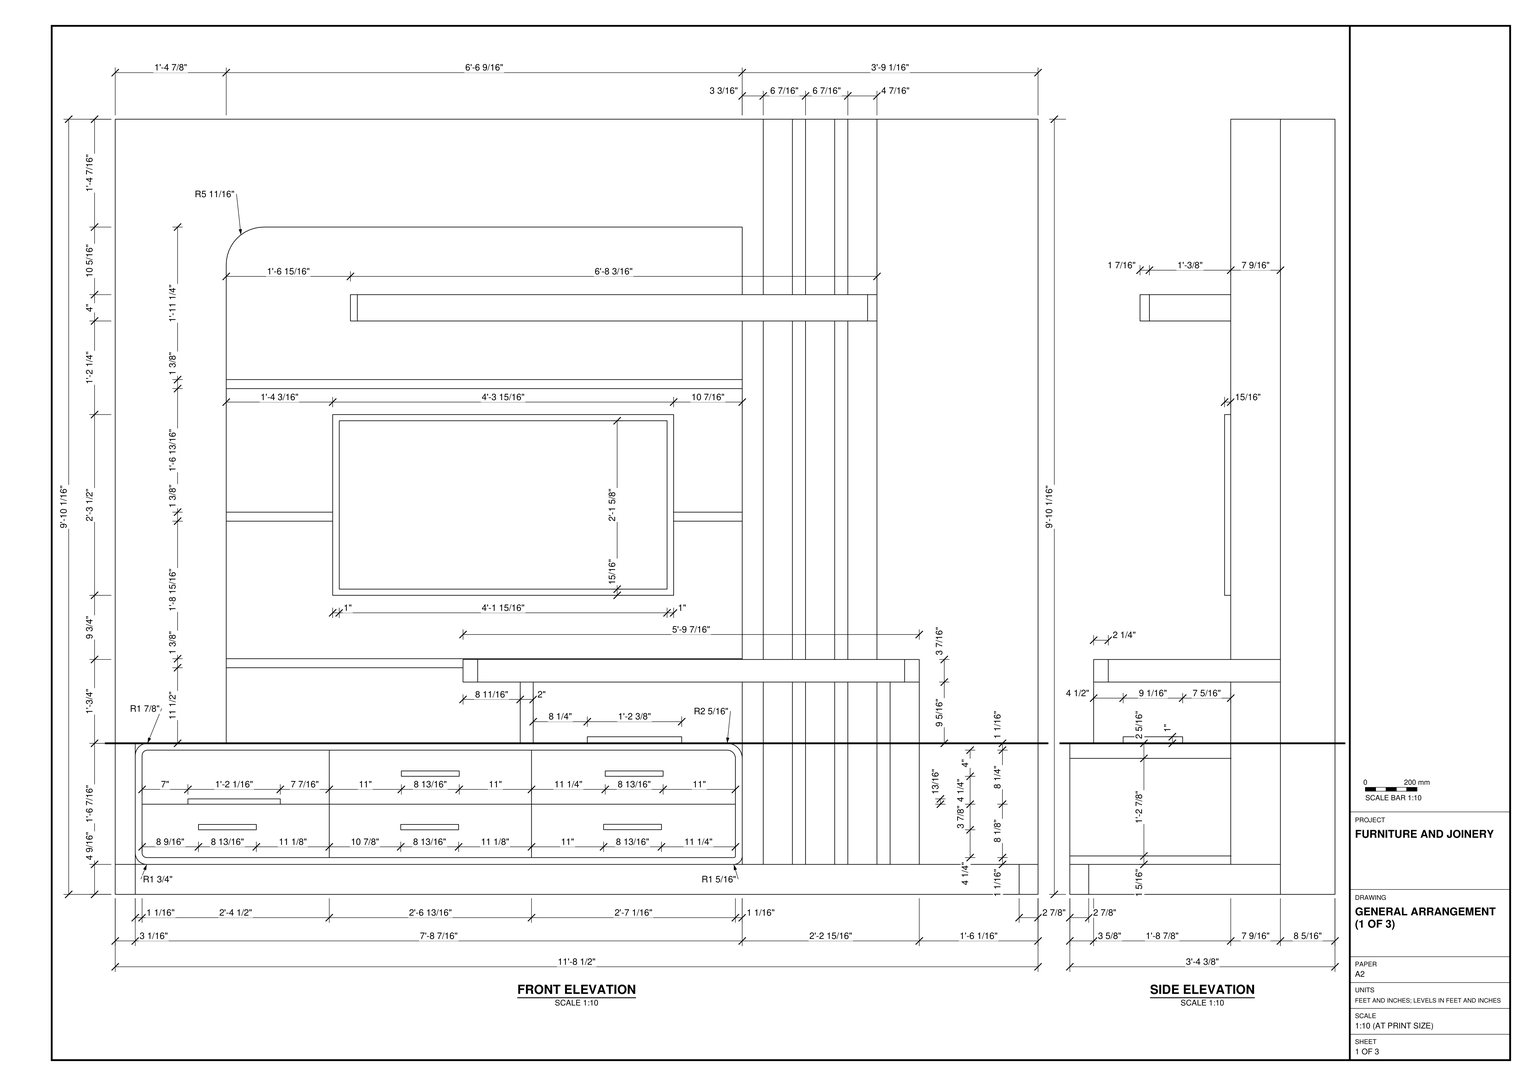
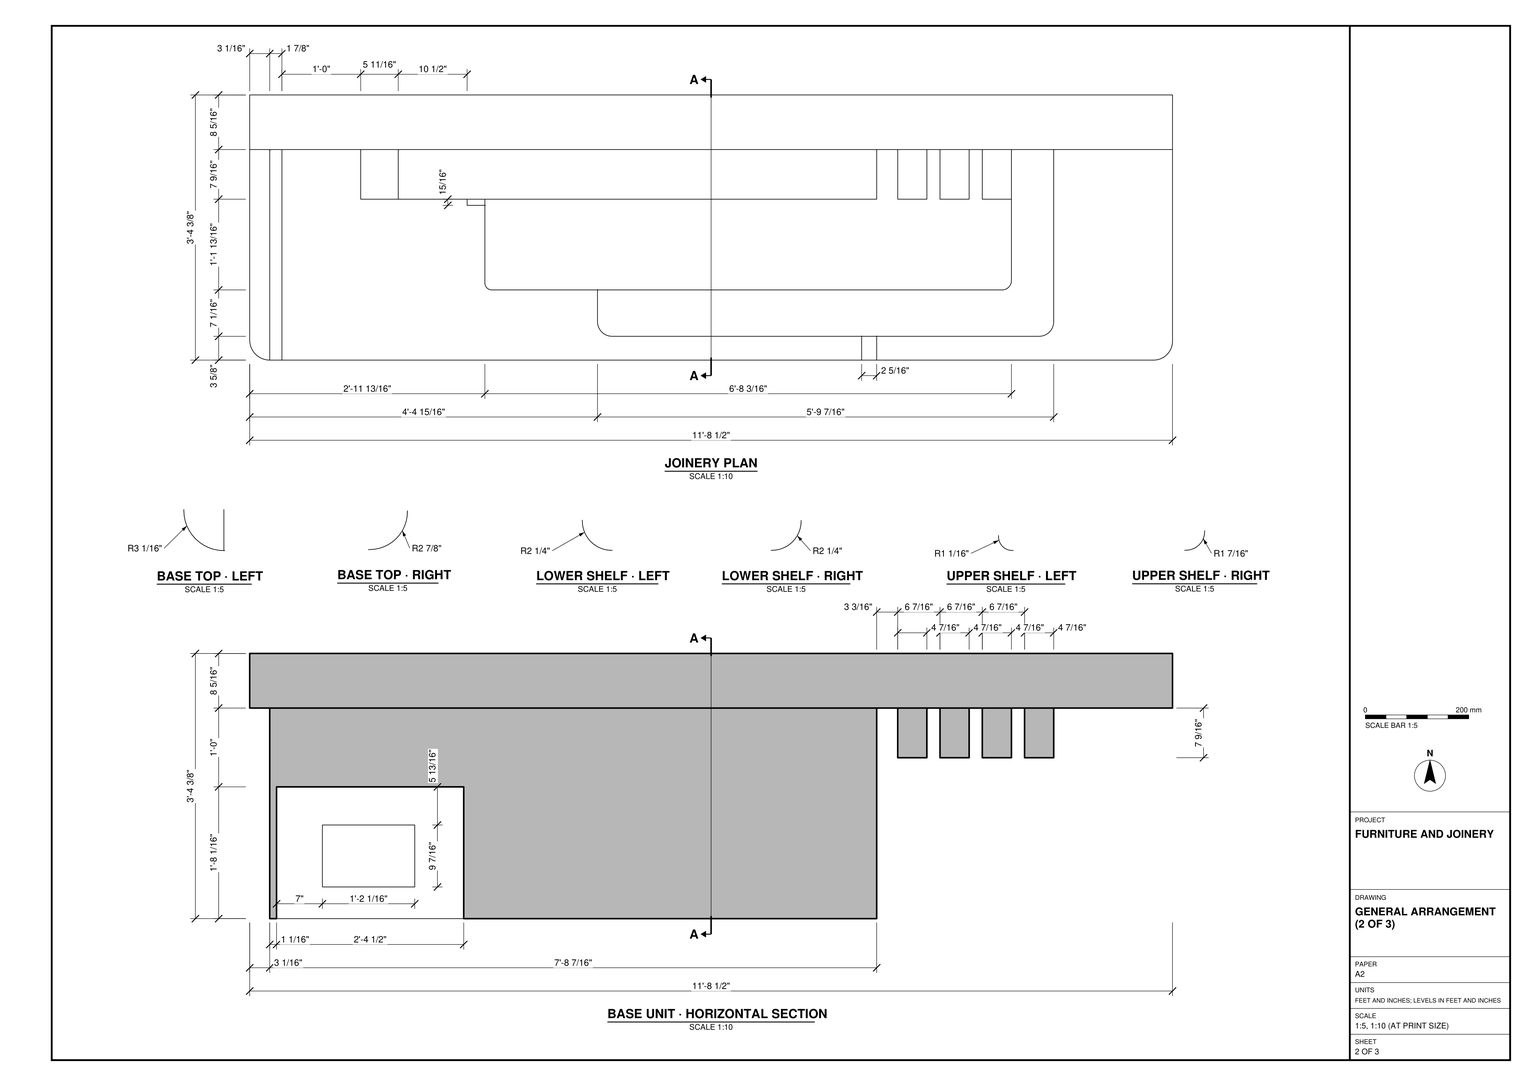
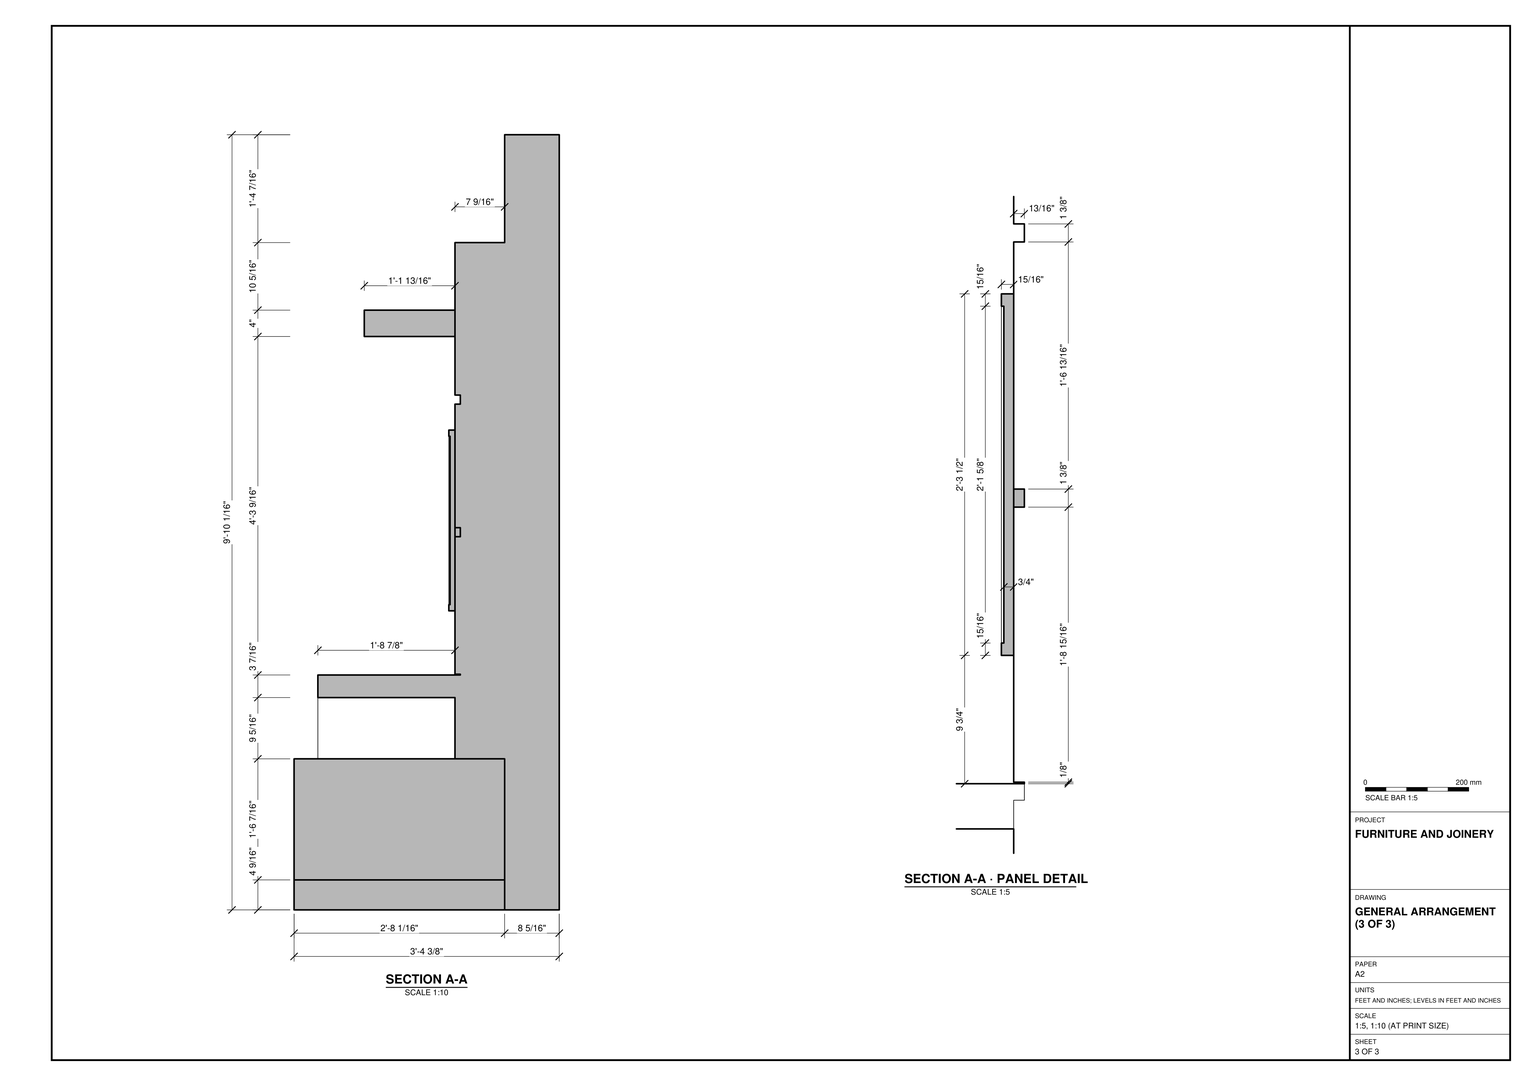
Build the media wall in SketchUp from task_files/diagram_01.pdf. Work in feet and inches. Use ±0'-0" as the floor datum and make the complete assembly 11'-8 1/2" wide, 3'-4 3/8" deep and 9'-10" high, including the rear wall.

Use the front elevation to lay out the raised backing panel, the framed screen, the narrow vertical strips on the right and the low storage cabinet on the left. Round the upper-left corner of the backing panel and form the horizontal grooves across its face. Set the screen between the two shelves. The upper shelf starts farther left, while the lower shelf extends farther right and projects farther forward. Use the plan and corner details to shape the front corners of the shelves and base top. Follow section A-A for the thickness of the rear wall, the changes in face depth and the clear space between the lower shelf and cabinet. Model the cabinet surround, bay divisions and pulls as shown in elevation.

Keep the rear wall and distinct joinery pieces in separate groups or components, and use components for repeated parts. Any decor or loose items shown may be represented by suitable library components. Save one SketchUp model as output_files/media_wall_with_base_storage_and_staggered_shelves.skp.

# SketchUp Ruby script. Lengths in inches.
U = 1.inch
M = Sketchup.active_model
def pt(a) = Geom::Point3d.new(a.map { |v| v * U })
def face(e, loops, mat)
  f = e.add_face(loops[0].map { |a| pt(a) })
  loops[1..].each { |l| e.add_face(l.map { |a| pt(a) }).erase! }
  f.material = f.back_material = mat if mat
  f
end
# faces: each face lists its corners as indices into pts; further lists are holes
def faces(e, pts, list, mat = nil) = list.each { |f| face(e, (f[0].is_a?(Array) ? f : [f]).map { |l| l.map { |i| pts[i] } }, mat) }
# xy, xz, yz: faces in a plane at the given z, y or x. An outline is a flat list of corners, or four numbers for a rectangle; further outlines are holes
def ring(l) = l.size == 4 ? [[l[0], l[1]], [l[2], l[1]], [l[2], l[3]], [l[0], l[3]]] : l.each_slice(2).to_a
def flat(e, list, mat, &to3) = list.each { |f| face(e, (f[0].is_a?(Array) ? f : [f]).map { |l| ring(l).map { |u, v| to3.(u, v) } }, mat) }
def xy(e, z, list, mat = nil) = flat(e, list, mat) { |x, y| [x, y, z] }
def xz(e, y, list, mat = nil) = flat(e, list, mat) { |x, z| [x, y, z] }
def yz(e, x, list, mat = nil) = flat(e, list, mat) { |y, z| [x, y, z] }
def lines(e, pts, list) = list.each { |a, b| e.add_line(pt(pts[a]), pt(pts[b])) }
# prism: a flat outline (further loops are holes) pulled along v
def prism(e, loops, v, mat = nil)
  f = face(e, loops, mat); d = Geom::Vector3d.new(v.map { |x| x * U })
  f.pushpull(f.normal.samedirection?(d) ? d.length : -d.length)
end
def box(e, o, s, mat = nil) = prism(e, [[o, [o[0] + s[0], o[1], o[2]], [o[0] + s[0], o[1] + s[1], o[2]], [o[0], o[1] + s[1], o[2]]]], [0, 0, s[2]], mat)
def at(x, y, z, deg = 0) = Geom::Transformation.translation(pt([x, y, z])) * Geom::Transformation.rotation(ORIGIN, Z_AXIS, deg.degrees)
def axes(o, x, y, z) = Geom::Transformation.new([*x, 0, *y, 0, *z, 0, *pt(o).to_a, 1])
def part(name) = M.definitions.add(name)
# library, detail: a bought-in or finely detailed component or shape, given as its bounding box
def library(name, o, s) = part(name).tap { |d| box(d.entities, o, s) }
def detail(e, o, s) = box(e.add_group.entities, o, s)
def put(e, d, t, mat = nil) = e.add_instance(d, t).tap { |i| i.material = mat if mat }
def group(e, t, mat = nil) = e.add_group.tap { |g| g.transformation = t; g.material = mat if mat }.entities
root = M.entities
M.materials.add("[Carrera Marble]").color = [177, 149, 108]
M.materials.add("[Color C02]").color = [255, 204, 153]
M.materials.add("[Color D01]").color = [255, 242, 204]
M.materials.add("[Color M09]").color = [0, 0, 0]
M.materials.add("[Wood Cherry Original]").color = [152, 86, 42]
xy(root,18.35,[[3.05,0,2.65,0.03,2.26,0.1,1.88,0.23,1.53,0.41,1.19,0.63,0.89,0.89,0.63,1.19,0.41,1.53,0.23,1.88,0.1,2.26,0.03,2.65,0,3.05,0,32.0625,140.5,32.0625,140.5,2.88,140.48,2.5,140.4,2.13,140.28,1.78,140.11,1.44,139.9,1.125,139.66,0.84,139.375,0.6,139.06,0.39,138.72,0.22,138.37,0.1,138,0.02,137.62,0],[0,32.0625,140.5,40.375]])
xy(root,22.91,[[3.05,0,3.05,32.0625,0,32.0625,0,3.05,0.03,2.65,0.1,2.26,0.23,1.88,0.41,1.53,0.63,1.19,0.89,0.89,1.19,0.63,1.53,0.41,1.88,0.23,2.26,0.1,2.65,0.03],[3.05,0,4.8,31.9375],[4.8,0,4.8,31.9375,3.05,31.9375,3.05,32.0625,94.17,32.0625,94.17,0],[94.17,0,95.46,32.0625],[98.66,24.5,103.1,32.0625],
  [105.1,24.5,109.54,32.0625],[111.54,24.5,115.98,32.0625],[117.98,24.5,122.41,32.0625]])
xy(root,22.91,[[95.46,0,137.62,0,138,0.02,138.37,0.1,138.72,0.22,139.06,0.39,139.375,0.6,139.66,0.84,139.9,1.125,140.11,1.44,140.28,1.78,140.4,2.13,140.48,2.5,140.5,2.88,140.5,32.0625,122.41,32.0625,122.41,24.5,117.98,24.5,117.98,32.0625,115.98,32.0625,115.98,24.5,111.54,24.5,111.54,32.0625,109.54,32.0625,109.54,24.5,105.1,24.5,105.1,32.0625,103.1,32.0625,103.1,24.5,98.66,24.5,98.66,32.0625,95.46,32.0625]],"[Color D01]")
xy(root,32.08,[[[4.09,0,32.59,20.0625],[11.07,4.82,25.13,14.26]]],"[Color D01]")
xy(root,32.89,[[11.07,4.82,25.13,14.26]],"[Color M09]")
xy(root,40.3125,[[4.91,0,32.59,20.0625]],"[Color D01]")
xy(root,41.35,[[16.9,24.5,93.17,32.0625],[93.17,24.5,95.46,32.0625]])
xy(root,41.35,[[[4.91,0,93.17,0,93.17,24.5,63.64,24.5,63.64,3.625,61.66,3.625,61.66,24.5,16.9,24.5,16.9,32.0625,4.91,32.0625],[71.87,8.12,86.25,17.18]]],"[Color D01]")
xy(root,42.35,[[71.87,8.12,86.25,17.18]],"[Color M09]")
xy(root,50.67,[[55.18,3.625,54.89,3.64,54.61,3.7,54.33,3.79,54.07,3.92,53.83,4.09,53.61,4.28,53.41,4.5,53.25,4.74,53.12,5,53.03,5.28,52.97,5.5625,52.95,5.86,52.95,24.5,61.66,24.5,61.66,3.625],[61.66,3.625,63.64,24.5],[98.66,24.5,103.1,26.8125],[105.1,24.5,109.54,26.8125],[111.54,24.5,115.98,26.8125],
  [117.98,24.5,122.41,32.0625]])
xy(root,50.67,[[63.64,3.625,63.64,24.5,95.46,24.5,95.46,32.0625,98.66,32.0625,98.66,24.5,103.1,24.5,103.1,32.0625,105.1,32.0625,105.1,24.5,109.54,24.5,109.54,32.0625,111.54,32.0625,111.54,24.5,115.98,24.5,115.98,32.0625,117.98,32.0625,117.98,24.5,122.41,24.5,122.41,5.86,122.39,5.5625,122.34,5.28,122.24,5,122.11,4.74,121.95,4.5,121.76,4.28,121.54,4.09,121.3,3.92,121.04,3.79,120.76,3.7,120.47,3.64,120.18,3.625]],"[Color D01]")
xy(root,52.86,[[16.9,24.5,52.95,25.3125]])
xy(root,54.12,[[98.66,24.5,103.1,26.8125],[105.1,24.5,109.54,26.8125],[111.54,24.5,115.98,26.8125]])
xy(root,54.12,[[55.18,3.625,120.18,3.625,120.47,3.64,120.76,3.7,121.04,3.79,121.3,3.92,121.54,4.09,121.76,4.28,121.95,4.5,122.11,4.74,122.24,5,122.34,5.28,122.39,5.5625,122.41,5.86,122.41,32.0625,115.98,32.0625,115.98,24.5,111.54,24.5,111.54,32.0625,109.54,32.0625,109.54,24.5,105.1,24.5,105.1,32.0625,103.1,32.0625,103.1,24.5,98.66,24.5,98.66,32.0625,95.46,32.0625,95.46,25.3125,52.95,25.3125,52.95,5.86,52.97,5.5625,53.03,5.28,53.12,5,53.25,4.74,53.41,4.5,53.61,4.28,53.83,4.09,54.07,3.92,54.33,3.79,54.61,3.7,54.89,3.64]],"[Color D01]")
xy(root,54.23,[[16.9,24.5,95.46,25.3125]])
xy(root,75.17,[[16.9,24.5,95.46,25.3125]])
xy(root,76.55,[[16.9,24.5,95.46,25.3125]])
xy(root,95.36,[[16.9,24.5,95.46,25.3125]])
xy(root,96.73,[[16.9,24.5,95.46,25.3125]])
xy(root,105.65,[[36.86,10.6875,36.72,10.7,36.59,10.72,36.46,10.77,36.33,10.83,36.22,10.91,36.12,11,36.03,11.1,35.95,11.21,35.89,11.34,35.84,11.47,35.82,11.6,35.81,11.74,35.81,24.5,95.46,24.5,95.46,32.0625,98.66,32.0625,98.66,24.5,103.1,24.5,103.1,35.125,105.1,35.125,105.1,24.5,109.54,24.5,109.54,35.125,111.54,35.125,111.54,24.5,115.98,24.5,115.98,12.11,115.96,11.93,115.93,11.74,115.87,11.57,115.78,11.4,115.68,11.25,115.56,11.11,115.42,10.98,115.26,10.88,115.1,10.8,114.92,10.74,114.74,10.7,114.55,10.6875]])
xy(root,109.67,[[36.86,10.6875,114.55,10.6875,114.74,10.7,114.92,10.74,115.1,10.8,115.26,10.88,115.42,10.98,115.56,11.11,115.68,11.25,115.78,11.4,115.87,11.57,115.93,11.74,115.96,11.93,115.98,12.11,115.98,24.5,111.54,24.5,111.54,35.125,109.54,35.125,109.54,24.5,105.1,24.5,105.1,35.125,103.1,35.125,103.1,24.5,98.66,24.5,98.66,32.0625,95.46,32.0625,95.46,24.5,35.81,24.5,35.81,11.74,35.82,11.6,35.84,11.47,35.89,11.34,35.95,11.21,36.03,11.1,36.12,11,36.22,10.91,36.33,10.83,36.46,10.77,36.59,10.72,36.72,10.7]],"[Color D01]")
xy(root,119.95,[[22.62,24.5,95.46,32.0625]],"[Color D01]")
xy(root,136.38,[[0,32.0625,140.5,40.375]],"[Color D01]")
xy(root,136.38,[[98.66,24.5,103.1,32.0625],[105.1,24.5,109.54,32.0625],[111.54,24.5,115.98,32.0625]],"[Wood Cherry Original]")
xz(root,0,[[3.05,18.35,137.62,22.91],[[4.8,22.91,94.17,22.91,94.34,22.92,94.51,22.96,94.67,23.01,94.82,23.08,94.96,23.18,95.08,23.29,95.2,23.42,95.29,23.56,95.36,23.71,95.42,23.87,95.45,24.03,95.46,24.2,95.46,39.06,95.44,39.36,95.38,39.65,95.29,39.94,95.15,40.2,94.99,40.45,94.79,40.68,94.56,40.875,94.32,41.04,94.05,41.18,93.76,41.27,93.47,41.33,93.17,41.35,4.91,41.35,4.67,41.33,4.43,41.29,4.2,41.21,3.98,41.1,3.78,40.97,3.59,40.81,3.43,40.62,3.3,40.42,3.19,40.2,3.11,39.97,3.07,39.73,3.05,39.49,3.05,24.66,3.07,24.43,3.11,24.21,3.18,23.99,3.28,23.79,3.41,23.6,3.5625,23.42,3.73,23.27,3.92,23.15,4.13,23.05,4.35,22.97,4.57,22.93],[4.8,23.95,4.62,23.97,4.53,24,4.44,24.04,4.3,24.16,4.23,24.23,4.18,24.31,4.14,24.39,4.11,24.48,4.09,24.57,4.09,39.6,4.12,39.7,4.15,39.81,4.2,39.9,4.26,39.99,4.33,40.07,4.41,40.14,4.5,40.2,4.59,40.25,4.7,40.28,4.8,40.31,4.91,40.3125,93.17,40.3125,93.33,40.3,93.49,40.27,93.65,40.22,93.8,40.14,93.93,40.05,94.06,39.95,94.17,39.82,94.26,39.69,94.33,39.54,94.38,39.38,94.41,39.22,94.42,39.06,94.42,24.14,94.41,24.1,94.39,24.07,94.37,24.05,94.35,24.02,94.33,24,94.3,23.98,94.21,23.95]]],"[Color D01]")
xz(root,0,[[12.67,28.18,21.48,28.99],[43.47,28.18,52.28,28.99],[74.35,28.2,83.17,29.01],[43.5625,36.33,52.375,37.14],[74.61,36.33,83.42,37.14]],"[Color M09]")
xz(root,0,[[[4.8,23.95,32.59,23.95,32.59,32.08,4.09,32.08,4.09,24.57,4.11,24.48,4.14,24.39,4.18,24.31,4.23,24.23,4.3,24.16,4.44,24.04,4.53,24,4.62,23.97],[12.67,28.18,21.48,28.99]],[[32.59,23.95,63.38,32.08],[43.47,28.18,52.28,28.99]],[[63.38,23.95,94.21,23.95,94.3,23.98,94.33,24,94.35,24.02,94.37,24.05,94.39,24.07,94.41,24.1,94.42,24.14,94.42,32.08,63.38,32.08],[74.35,28.2,83.17,29.01]],[[32.59,32.08,63.38,40.3125],[43.5625,36.33,52.375,37.14]],[[63.38,32.08,94.42,32.08,94.42,39.06,94.41,39.22,94.38,39.38,94.33,39.54,94.26,39.69,94.17,39.82,94.06,39.95,93.93,40.05,93.8,40.14,93.65,40.22,93.49,40.27,93.33,40.3,93.17,40.3125,63.38,40.3125],[74.61,36.33,83.42,37.14]]],"[Wood Cherry Original]")
xz(root,3.625,[[61.66,41.35,63.64,50.67],[55.18,50.67,120.18,54.12]],"[Color D01]")
xz(root,4.82,[[11.07,32.08,25.13,32.89]],"[Color M09]")
xz(root,8.12,[[71.87,41.35,86.25,42.35]],"[Color M09]")
xz(root,10.6875,[[36.86,105.65,114.55,109.67]],"[Color D01]")
xz(root,14.26,[[11.07,32.08,25.13,32.89]])
xz(root,17.18,[[71.87,41.35,86.25,42.35]])
xz(root,20.0625,[[4.09,32.08,32.59,32.08,32.59,40.3125,4.91,40.3125,4.8,40.31,4.7,40.28,4.59,40.25,4.5,40.2,4.41,40.14,4.33,40.07,4.26,39.99,4.2,39.9,4.15,39.81,4.12,39.7,4.09,39.6]],"[Color D01]")
xz(root,24.5,[[61.66,41.35,63.64,50.67],[35.81,105.65,95.46,109.67],[98.66,105.65,103.1,109.67],[105.1,105.65,109.54,109.67],[111.54,105.65,115.98,109.67]])
xz(root,24.5,[[16.9,41.35,61.66,41.35,61.66,50.67,52.95,50.67,52.95,52.86,16.9,52.86],[16.9,54.23,95.46,75.17],[16.9,76.55,95.46,95.36],[16.9,96.73,95.46,96.73,95.46,105.65,35.81,105.65,35.81,109.67,95.46,109.67,95.46,119.95,22.62,119.95,21.87,119.9,21.14,119.76,20.43,119.52,19.76,119.1875,19.14,118.77,18.57,118.28,18.08,117.72,17.66,117.09,17.33,116.42,17.09,115.71,16.95,114.98,16.9,114.23]],"[Carrera Marble]")
xz(root,24.5,[[63.64,41.35,95.46,50.67]],"[Color D01]")
xz(root,24.5,[[98.66,22.91,103.1,50.67],[105.1,22.91,109.54,50.67],[111.54,22.91,115.98,50.67],[117.98,22.91,122.41,50.67],[98.66,54.12,103.1,105.65],
  [105.1,54.12,109.54,105.65],[111.54,54.12,115.98,105.65],[98.66,109.67,103.1,136.38],[105.1,109.67,109.54,136.38],[111.54,109.67,115.98,136.38]],"[Wood Cherry Original]")
xz(root,25.3125,[[16.9,52.86,52.95,52.86,52.95,54.12,95.46,54.12,95.46,54.23,16.9,54.23],[16.9,75.17,95.46,76.55],[16.9,95.36,95.46,96.73]],"[Color M09]")
xz(root,26.8125,[[98.66,50.67,103.1,54.12],[105.1,50.67,109.54,54.12],[111.54,50.67,115.98,54.12]])
xz(root,31.9375,[[3.05,22.91,4.8,22.91,4.57,22.93,4.35,22.97,4.13,23.05,3.92,23.15,3.73,23.27,3.5625,23.42,3.41,23.6,3.28,23.79,3.18,23.99,3.11,24.21,3.07,24.43,3.05,24.66]])
xz(root,32.0625,[[0,18.35,140.5,22.91],[3.05,22.91,16.9,22.91,16.9,41.35,4.91,41.35,4.67,41.33,4.43,41.29,4.2,41.21,3.98,41.1,3.78,40.97,3.59,40.81,3.43,40.62,3.3,40.42,3.19,40.2,3.11,39.97,3.07,39.73,3.05,39.49],[16.9,22.91,94.17,22.91,94.34,22.92,94.51,22.96,94.67,23.01,94.82,23.08,94.96,23.18,95.08,23.29,95.2,23.42,95.29,23.56,95.36,23.71,95.42,23.87,95.45,24.03,95.46,24.2,95.46,39.06,95.44,39.36,95.38,39.65,95.29,39.94,95.15,40.2,94.99,40.45,94.79,40.68,94.56,40.875,94.32,41.04,94.05,41.18,93.76,41.27,93.47,41.33,93.17,41.35,16.9,41.35],[95.46,22.91,98.66,50.67],[98.66,22.91,103.1,136.38],
  [103.1,22.91,105.1,50.67],[105.1,22.91,109.54,136.38],[109.54,22.91,111.54,50.67],[111.54,22.91,115.98,136.38],[115.98,22.91,117.98,50.67],
  [117.98,22.91,122.41,50.67],[103.1,50.67,105.1,54.12],[109.54,50.67,111.54,54.12],[115.98,50.67,122.41,54.12],[95.46,54.12,98.66,105.65],
  [103.1,54.12,105.1,136.38],[109.54,54.12,111.54,136.38],[95.46,105.65,98.66,109.67]])
xz(root,32.0625,[[0,22.91,3.05,22.91,3.05,41.35,16.9,41.35,16.9,114.23,16.95,114.98,17.09,115.71,17.33,116.42,17.66,117.09,18.08,117.72,18.57,118.28,19.14,118.77,19.76,119.1875,20.43,119.52,21.14,119.76,21.87,119.9,22.62,119.95,95.46,119.95,95.46,109.67,98.66,109.67,98.66,136.38,0,136.38],[122.41,22.91,140.5,22.91,140.5,136.38,115.98,136.38,115.98,54.12,122.41,54.12]],"[Color C02]")
xz(root,35.125,[[103.1,105.65,105.1,109.67],[109.54,105.65,111.54,109.67]])
xz(root,40.375,[[0,18.35,140.5,136.38]],"[Color D01]")
yz(root,0,[[3.05,18.35,32.0625,22.91],[32.0625,18.35,40.375,136.38]],"[Color D01]")
yz(root,3.05,[[31.9375,22.91,31.9375,24.66,0,24.66,0,39.49,32.0625,39.49,32.0625,22.91]],"[Color D01]")
yz(root,4.09,[[0,32.08,20.0625,39.49],[0,39.49,20.0625,39.6]],"[Color D01]")
yz(root,11.07,[[4.82,32.08,14.26,32.89]],"[Color M09]")
yz(root,16.9,[[24.5,41.35,24.5,52.86,25.3125,52.86,25.3125,54.23,24.5,54.23,24.5,75.17,25.3125,75.17,25.3125,76.55,24.5,76.55,24.5,95.36,25.3125,95.36,25.3125,96.73,24.5,96.73,24.5,114.23,32.0625,114.23,32.0625,41.35]],"[Color D01]")
yz(root,25.13,[[4.82,32.08,14.26,32.89]],"[Color M09]")
yz(root,32.59,[[0,32.08,20.0625,40.3125]],"[Color D01]")
yz(root,35.81,[[11.74,105.65,24.5,109.67]],"[Color D01]")
yz(root,52.95,[[5.86,50.67,5.86,54.12,25.3125,54.12,25.3125,52.86,24.5,52.86,24.5,50.67]],"[Color D01]")
yz(root,61.66,[[3.625,41.35,24.5,50.67]],"[Color D01]")
yz(root,63.64,[[3.625,41.35,24.5,50.67]],"[Color D01]")
yz(root,71.87,[[8.12,41.35,17.18,42.35]],"[Color M09]")
yz(root,86.25,[[8.12,41.35,17.18,42.35]],"[Color M09]")
yz(root,95.46,[[24.5,105.65,32.0625,109.67]])
yz(root,95.46,[[25.3125,54.12,32.0625,54.12,32.0625,105.65,24.5,105.65,24.5,96.73,25.3125,96.73,25.3125,95.36,24.5,95.36,24.5,76.55,25.3125,76.55,25.3125,75.17,24.5,75.17,24.5,54.23,25.3125,54.23],[24.5,109.67,32.0625,119.95]],"[Color C02]")
yz(root,95.46,[[0,24.2,32.0625,39.06],[24.5,41.35,32.0625,50.67]],"[Color D01]")
yz(root,98.66,[[26.8125,50.67,32.0625,54.12],[24.5,105.65,32.0625,109.67]])
yz(root,98.66,[[24.5,22.91,32.0625,50.67],[24.5,54.12,32.0625,105.65],[24.5,109.67,32.0625,136.38]],"[Wood Cherry Original]")
yz(root,103.1,[[26.8125,50.67,32.0625,54.12],[24.5,105.65,32.0625,109.67],[32.0625,105.65,35.125,109.67]])
yz(root,103.1,[[24.5,22.91,32.0625,50.67],[24.5,54.12,32.0625,105.65],[24.5,109.67,32.0625,136.38]],"[Wood Cherry Original]")
yz(root,105.1,[[26.8125,50.67,32.0625,54.12],[24.5,105.65,32.0625,109.67],[32.0625,105.65,35.125,109.67]])
yz(root,105.1,[[24.5,22.91,32.0625,50.67],[24.5,54.12,32.0625,105.65],[24.5,109.67,32.0625,136.38]],"[Wood Cherry Original]")
yz(root,109.54,[[26.8125,50.67,32.0625,54.12],[24.5,105.65,32.0625,109.67],[32.0625,105.65,35.125,109.67]])
yz(root,109.54,[[24.5,22.91,32.0625,50.67],[24.5,54.12,32.0625,105.65],[24.5,109.67,32.0625,136.38]],"[Wood Cherry Original]")
yz(root,111.54,[[26.8125,50.67,32.0625,54.12],[24.5,105.65,32.0625,109.67],[32.0625,105.65,35.125,109.67]])
yz(root,111.54,[[24.5,22.91,32.0625,50.67],[24.5,54.12,32.0625,105.65],[24.5,109.67,32.0625,136.38]],"[Wood Cherry Original]")
yz(root,115.98,[[26.8125,50.67,32.0625,54.12]])
yz(root,115.98,[[12.11,105.65,24.5,109.67]],"[Color D01]")
yz(root,115.98,[[24.5,22.91,32.0625,50.67],[24.5,54.12,32.0625,136.38]],"[Wood Cherry Original]")
yz(root,117.98,[[24.5,22.91,32.0625,50.67]],"[Wood Cherry Original]")
yz(root,122.41,[[5.86,50.67,32.0625,54.12]],"[Color D01]")
yz(root,122.41,[[24.5,22.91,32.0625,50.67]],"[Wood Cherry Original]")
yz(root,140.5,[[2.88,18.35,32.0625,22.91],[32.0625,18.35,40.375,136.38]],"[Color D01]")
p = [[2.65,0.03,22.91],[2.26,0.1,22.91],[2.26,0.1,18.35],[2.65,0.03,18.35],[3.05,0,22.91],[3.05,0,18.35],
  [138,0.02,22.91],[137.62,0,22.91],[137.62,0,18.35],[138,0.02,18.35],[138.37,0.1,22.91],[138.37,0.1,18.35],
  [1.88,0.23,22.91],[1.88,0.23,18.35],[138.72,0.22,22.91],[138.72,0.22,18.35],[1.53,0.41,22.91],[1.53,0.41,18.35],
  [139.06,0.39,22.91],[139.06,0.39,18.35],[1.19,0.63,22.91],[1.19,0.63,18.35],[139.375,0.6,22.91],[139.375,0.6,18.35],
  [0.89,0.89,22.91],[0.89,0.89,18.35],[139.66,0.84,22.91],[139.66,0.84,18.35],[139.9,1.125,22.91],[139.9,1.125,18.35],
  [0.63,1.19,22.91],[0.63,1.19,18.35],[140.11,1.44,22.91],[140.11,1.44,18.35],[0.41,1.53,22.91],[0.41,1.53,18.35],
  [140.28,1.78,22.91],[140.28,1.78,18.35],[0.23,1.88,22.91],[0.23,1.88,18.35],[140.4,2.13,22.91],[140.4,2.13,18.35],
  [0.1,2.26,22.91],[0.1,2.26,18.35],[140.48,2.5,22.91],[140.48,2.5,18.35],[0.03,2.65,22.91],[0.03,2.65,18.35],
  [140.5,2.88,22.91],[140.5,2.88,18.35],[0,3.05,22.91],[0,3.05,18.35],[4.57,0,22.93],[4.35,0,22.97],
  [4.35,31.9375,22.97],[4.57,31.9375,22.93],[4.8,0,22.91],[4.8,31.9375,22.91],[94.34,0,22.92],[94.17,0,22.91],
  [94.17,32.0625,22.91],[94.34,32.0625,22.92],[94.51,0,22.96],[94.51,32.0625,22.96],[4.13,0,23.05],[3.92,0,23.15],
  [3.92,31.9375,23.15],[4.13,31.9375,23.05],[94.67,0,23.01],[94.67,32.0625,23.01],[94.82,0,23.08],[94.82,32.0625,23.08],
  [3.73,0,23.27],[3.73,31.9375,23.27],[94.96,0,23.18],[94.96,32.0625,23.18],[95.08,0,23.29],[95.08,32.0625,23.29],
  [3.5625,0,23.42],[3.5625,31.9375,23.42],[95.2,0,23.42],[95.2,32.0625,23.42],[3.41,0,23.6],[3.41,31.9375,23.6],
  [95.29,0,23.56],[95.29,32.0625,23.56],[3.28,0,23.79],[3.28,31.9375,23.79],[95.36,0,23.71],[95.36,32.0625,23.71],
  [95.42,0,23.87],[95.42,32.0625,23.87],[3.18,0,23.99],[3.18,31.9375,23.99],[95.45,0,24.03],[95.45,32.0625,24.03],
  [3.11,0,24.21],[3.11,31.9375,24.21],[95.46,0,24.2],[95.46,32.0625,24.2],[3.07,0,24.43],[3.07,31.9375,24.43],
  [3.05,0,24.66],[3.05,31.9375,24.66],[95.44,0,39.36],[95.46,0,39.06],[95.46,32.0625,39.06],[95.44,32.0625,39.36],
  [95.38,0,39.65],[95.38,32.0625,39.65],[3.05,0,39.49],[3.07,0,39.73],[3.07,32.0625,39.73],[3.05,32.0625,39.49],
  [4.12,0,39.7],[4.09,0,39.6],[4.09,20.0625,39.6],[4.12,20.0625,39.7],[3.11,0,39.97],[3.11,32.0625,39.97],
  [4.15,0,39.81],[4.15,20.0625,39.81],[95.29,0,39.94],[95.29,32.0625,39.94],[4.2,0,39.9],[4.2,20.0625,39.9],
  [4.26,0,39.99],[4.26,20.0625,39.99],[95.15,0,40.2],[95.15,32.0625,40.2],[3.19,0,40.2],[3.19,32.0625,40.2],
  [4.33,0,40.07],[4.33,20.0625,40.07],[4.41,0,40.14],[4.41,20.0625,40.14],[4.5,0,40.2],[4.5,20.0625,40.2],
  [3.3,0,40.42],[3.3,32.0625,40.42],[4.59,0,40.25],[4.59,20.0625,40.25],[4.7,0,40.28],[4.7,20.0625,40.28],
  [94.99,0,40.45],[94.99,32.0625,40.45],[4.8,0,40.31],[4.8,20.0625,40.31],[4.91,0,40.3125],[4.91,20.0625,40.3125],
  [3.43,0,40.62],[3.43,32.0625,40.62],[94.79,0,40.68],[94.79,32.0625,40.68],[3.59,0,40.81],[3.59,32.0625,40.81],
  [94.56,0,40.875],[94.56,32.0625,40.875],[3.78,0,40.97],[3.78,32.0625,40.97],[94.32,0,41.04],[94.32,32.0625,41.04],
  [3.98,0,41.1],[3.98,32.0625,41.1],[94.05,0,41.18],[94.05,32.0625,41.18],[4.2,0,41.21],[4.2,32.0625,41.21],
  [4.43,0,41.29],[4.43,32.0625,41.29],[93.76,0,41.27],[93.76,32.0625,41.27],[4.67,0,41.33],[4.67,32.0625,41.33],
  [4.91,0,41.35],[4.91,32.0625,41.35],[93.17,0,41.35],[93.47,0,41.33],[93.47,32.0625,41.33],[93.17,32.0625,41.35],
  [93.17,24.5,41.35],[54.89,3.64,54.12],[54.61,3.7,54.12],[54.61,3.7,50.67],[54.89,3.64,50.67],[55.18,3.625,54.12],
  [55.18,3.625,50.67],[120.47,3.64,54.12],[120.18,3.625,54.12],[120.18,3.625,50.67],[120.47,3.64,50.67],[120.76,3.7,54.12],
  [120.76,3.7,50.67],[54.33,3.79,54.12],[54.33,3.79,50.67],[121.04,3.79,54.12],[121.04,3.79,50.67],[54.07,3.92,54.12],
  [54.07,3.92,50.67],[121.3,3.92,54.12],[121.3,3.92,50.67],[53.83,4.09,54.12],[53.83,4.09,50.67],[121.54,4.09,54.12],
  [121.54,4.09,50.67],[53.61,4.28,54.12],[53.61,4.28,50.67],[121.76,4.28,54.12],[121.76,4.28,50.67],[53.41,4.5,54.12],
  [53.41,4.5,50.67],[121.95,4.5,54.12],[121.95,4.5,50.67],[53.25,4.74,54.12],[53.25,4.74,50.67],[122.11,4.74,54.12],
  [122.11,4.74,50.67],[53.12,5,54.12],[53.12,5,50.67],[122.24,5,54.12],[122.24,5,50.67],[53.03,5.28,54.12],
  [53.03,5.28,50.67],[122.34,5.28,54.12],[122.34,5.28,50.67],[52.97,5.5625,54.12],[52.97,5.5625,50.67],[122.39,5.5625,54.12],
  [122.39,5.5625,50.67],[52.95,5.86,54.12],[52.95,5.86,50.67],[122.41,5.86,54.12],[122.41,5.86,50.67],[36.59,10.72,109.67],
  [36.46,10.77,109.67],[36.46,10.77,105.65],[36.59,10.72,105.65],[36.72,10.7,109.67],[36.72,10.7,105.65],[36.86,10.6875,109.67],
  [36.86,10.6875,105.65],[114.74,10.7,109.67],[114.55,10.6875,109.67],[114.55,10.6875,105.65],[114.74,10.7,105.65],[114.92,10.74,109.67],
  [114.92,10.74,105.65],[115.1,10.8,109.67],[115.1,10.8,105.65],[36.33,10.83,109.67],[36.22,10.91,109.67],[36.22,10.91,105.65],
  [36.33,10.83,105.65],[115.26,10.88,109.67],[115.26,10.88,105.65],[36.12,11,109.67],[36.12,11,105.65],[115.42,10.98,109.67],
  [115.42,10.98,105.65],[36.03,11.1,109.67],[36.03,11.1,105.65],[115.56,11.11,109.67],[115.56,11.11,105.65],[35.95,11.21,109.67],
  [35.95,11.21,105.65],[115.68,11.25,109.67],[115.68,11.25,105.65],[35.89,11.34,109.67],[35.89,11.34,105.65],[115.78,11.4,109.67],
  [115.78,11.4,105.65],[35.84,11.47,109.67],[35.84,11.47,105.65],[115.87,11.57,109.67],[115.87,11.57,105.65],[35.82,11.6,109.67],
  [35.82,11.6,105.65],[35.81,11.74,109.67],[35.81,11.74,105.65],[115.93,11.74,109.67],[115.93,11.74,105.65],[115.96,11.93,109.67],
  [115.96,11.93,105.65],[115.98,12.11,109.67],[115.98,12.11,105.65],[16.95,32.0625,114.98],[16.9,32.0625,114.23],[16.9,24.5,114.23],
  [16.95,24.5,114.98],[17.09,32.0625,115.71],[17.09,24.5,115.71],[17.33,32.0625,116.42],[17.33,24.5,116.42],[17.66,32.0625,117.09],
  [17.66,24.5,117.09],[18.08,32.0625,117.72],[18.08,24.5,117.72],[18.57,32.0625,118.28],[18.57,24.5,118.28],[19.14,32.0625,118.77],
  [19.14,24.5,118.77],[19.76,32.0625,119.1875],[19.76,24.5,119.1875],[20.43,32.0625,119.52],[20.43,24.5,119.52],[21.14,32.0625,119.76],
  [21.14,24.5,119.76],[21.87,32.0625,119.9],[21.87,24.5,119.9],[22.62,32.0625,119.95],[22.62,24.5,119.95],[3.05,32.0625,22.91],
  [3.05,37.5,22.91],[52.95,24.5,52.86],[95.46,24.5,52.86]]
faces(root,p,[[0,1,2,3],[4,0,3,5],[6,7,8,9],[10,6,9,11],[1,12,13,2],[14,10,11,15],[12,16,17,13],[18,14,15,19],
  [16,20,21,17],[22,18,19,23],[20,24,25,21],[26,22,23,27],[28,26,27,29],[24,30,31,25],[32,28,29,33],[30,34,35,31],
  [36,32,33,37],[34,38,39,35],[40,36,37,41],[38,42,43,39],[44,40,41,45],[42,46,47,43],[48,44,45,49],[46,50,51,47],
  [52,53,54,55],[56,52,55,57],[58,59,60,61],[62,58,61,63],[64,65,66,67],[53,64,67,54],[68,62,63,69],[70,68,69,71],
  [65,72,73,66],[74,70,71,75],[76,74,75,77],[72,78,79,73],[80,76,77,81],[78,82,83,79],[84,80,81,85],[82,86,87,83],
  [88,84,85,89],[90,88,89,91],[86,92,93,87],[94,90,91,95],[92,96,97,93],[98,94,95,99],[96,100,101,97],[100,102,103,101],
  [104,105,106,107],[108,104,107,109],[110,111,112,113],[114,115,116,117],[111,118,119,112],[120,114,117,121],[122,108,109,123],[124,120,121,125],
  [126,124,125,127],[128,122,123,129],[118,130,131,119],[132,126,127,133],[134,132,133,135],[136,134,135,137],[130,138,139,131],[140,136,137,141],
  [142,140,141,143],[144,128,129,145],[146,142,143,147],[148,146,147,149],[138,150,151,139],[152,144,145,153],[150,154,155,151],[156,152,153,157],
  [154,158,159,155],[160,156,157,161],[158,162,163,159],[164,160,161,165],[162,166,167,163],[166,168,169,167],[170,164,165,171],[168,172,173,169],
  [172,174,175,173],[176,177,178,179,180],[177,170,171,178],[181,182,183,184],[185,181,184,186],[187,188,189,190],[191,187,190,192],[182,193,194,183],
  [195,191,192,196],[193,197,198,194],[199,195,196,200],[197,201,202,198],[203,199,200,204],[201,205,206,202],[207,203,204,208],[205,209,210,206],
  [211,207,208,212],[209,213,214,210],[215,211,212,216],[213,217,218,214],[219,215,216,220],[217,221,222,218],[223,219,220,224],[221,225,226,222],
  [227,223,224,228],[225,229,230,226],[231,227,228,232],[233,234,235,236],[237,233,236,238],[239,237,238,240],[241,242,243,244],[245,241,244,246],
  [247,245,246,248],[249,250,251,252],[234,249,252,235],[253,247,248,254],[250,255,256,251],[257,253,254,258],[255,259,260,256],[261,257,258,262],
  [259,263,264,260],[265,261,262,266],[263,267,268,264],[269,265,266,270],[267,271,272,268],[273,269,270,274],[271,275,276,272],[275,277,278,276],
  [279,273,274,280],[281,279,280,282],[283,281,282,284],[285,286,287,288],[289,285,288,290],[291,289,290,292],[293,291,292,294],[295,293,294,296],
  [297,295,296,298],[299,297,298,300],[301,299,300,302],[303,301,302,304],[305,303,304,306],[307,305,306,308],[309,307,308,310]],"[Color D01]")
lines(root,p,[[311,312],[313,314]])
g1 = group(root,at(33.11,23.5625,63.88),"[Color M09]")
xy(g1,0,[[0,0,51.91,0.9375]])
xy(g1,0.94,[[1,0,50.91,0.1875]])
xy(g1,26.58,[[1,0,50.91,0.1875]])
xy(g1,27.52,[[0,0,51.91,0.9375]])
xz(g1,0,[[[0,0,51.91,27.52],[1,0.94,50.91,26.58]]])
xz(g1,0.1875,[[1,0.94,50.91,26.58]])
xz(g1,0.9375,[[0,0,51.91,27.52]])
yz(g1,0,[[0,0,0.9375,27.52]])
yz(g1,1,[[0,0.94,0.1875,26.58]])
yz(g1,50.91,[[0,0.94,0.1875,26.58]])
yz(g1,51.91,[[0,0,0.9375,27.52]])
